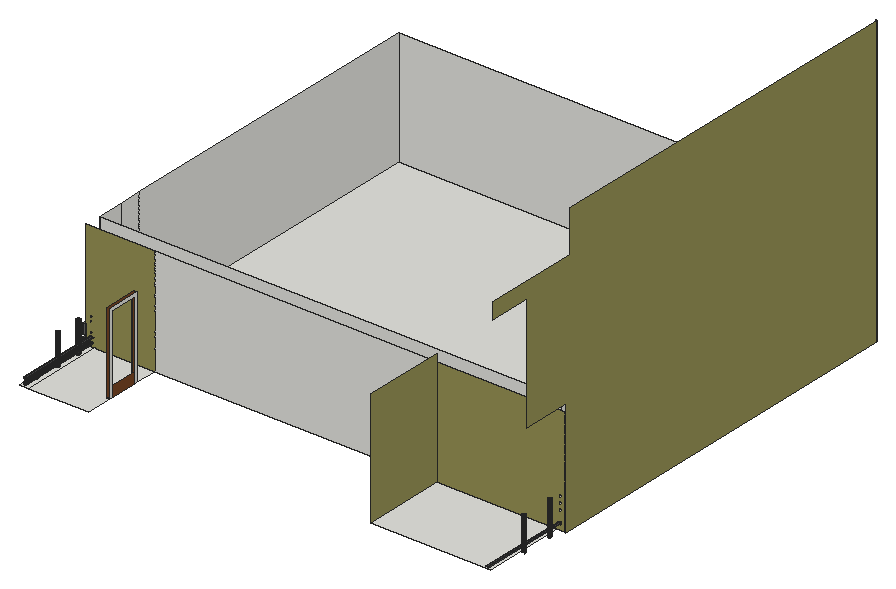
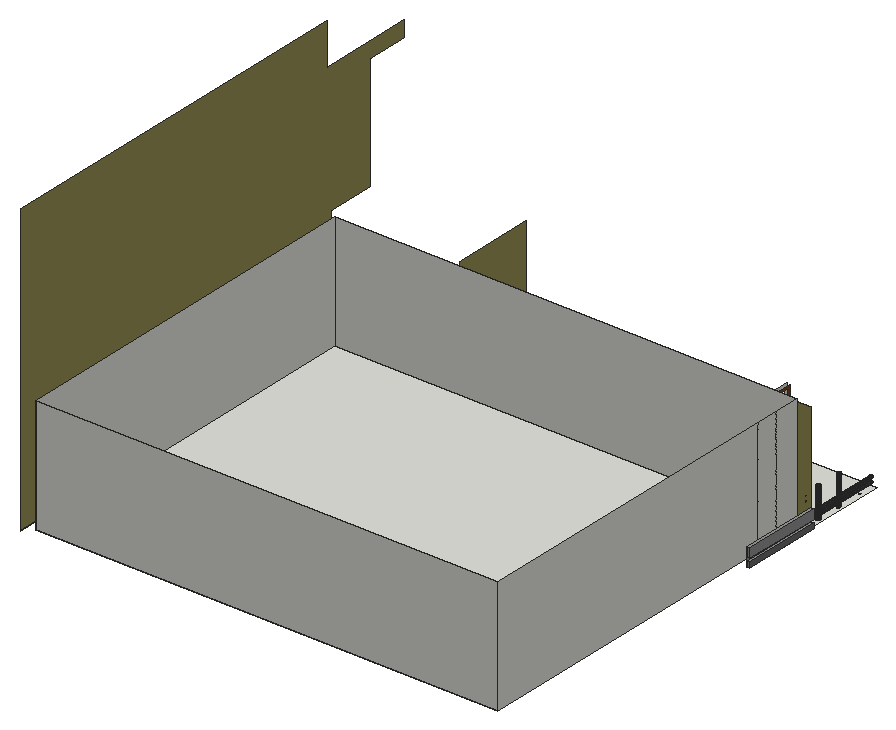
# SketchUp Ruby script. Lengths in inches.
U = 1.inch
M = Sketchup.active_model
def pt(a) = Geom::Point3d.new(a.map { |v| v * U })
def face(e, loops, mat)
  f = e.add_face(loops[0].map { |a| pt(a) })
  loops[1..].each { |l| e.add_face(l.map { |a| pt(a) }).erase! }
  f.material = f.back_material = mat if mat
  f
end
# faces: each face lists its corners as indices into pts; further lists are holes
def faces(e, pts, list, mat = nil) = list.each { |f| face(e, (f[0].is_a?(Array) ? f : [f]).map { |l| l.map { |i| pts[i] } }, mat) }
# xy, xz, yz: faces in a plane at the given z, y or x. An outline is a flat list of corners, or four numbers for a rectangle; further outlines are holes
def ring(l) = l.size == 4 ? [[l[0], l[1]], [l[2], l[1]], [l[2], l[3]], [l[0], l[3]]] : l.each_slice(2).to_a
def flat(e, list, mat, &to3) = list.each { |f| face(e, (f[0].is_a?(Array) ? f : [f]).map { |l| ring(l).map { |u, v| to3.(u, v) } }, mat) }
def xy(e, z, list, mat = nil) = flat(e, list, mat) { |x, y| [x, y, z] }
def xz(e, y, list, mat = nil) = flat(e, list, mat) { |x, z| [x, y, z] }
def yz(e, x, list, mat = nil) = flat(e, list, mat) { |y, z| [x, y, z] }
def lines(e, pts, list) = list.each { |a, b| e.add_line(pt(pts[a]), pt(pts[b])) }
# prism: a flat outline (further loops are holes) pulled along v
def prism(e, loops, v, mat = nil)
  f = face(e, loops, mat); d = Geom::Vector3d.new(v.map { |x| x * U })
  f.pushpull(f.normal.samedirection?(d) ? d.length : -d.length)
end
def box(e, o, s, mat = nil) = prism(e, [[o, [o[0] + s[0], o[1], o[2]], [o[0] + s[0], o[1] + s[1], o[2]], [o[0], o[1] + s[1], o[2]]]], [0, 0, s[2]], mat)
def at(x, y, z, deg = 0) = Geom::Transformation.translation(pt([x, y, z])) * Geom::Transformation.rotation(ORIGIN, Z_AXIS, deg.degrees)
def axes(o, x, y, z) = Geom::Transformation.new([*x, 0, *y, 0, *z, 0, *pt(o).to_a, 1])
def part(name) = M.definitions.add(name)
# library, detail: a bought-in or finely detailed component or shape, given as its bounding box
def library(name, o, s) = part(name).tap { |d| box(d.entities, o, s) }
def detail(e, o, s) = box(e.add_group.entities, o, s)
def put(e, d, t, mat = nil) = e.add_instance(d, t).tap { |i| i.material = mat if mat }
def group(e, t, mat = nil) = e.add_group.tap { |g| g.transformation = t; g.material = mat if mat }.entities
root = M.entities
M.materials.add("[0057_DarkKhaki]").color = [150, 145, 85]
M.materials.add("[0134_DimGray]").color = [105, 105, 105]
M.materials.add("[0137_Black]").color = [71, 71, 71]
M.materials.add("[Color M05]").color = [145, 145, 145]
M.materials.add("[Wood Veneer 01]").color = [120, 70, 37]
xy(root,123,[[[11.875,31.0625,20.875,116.75],[15.96,45.8,15.46,45.87,15,46.06,14.59,46.37,14.29,46.77,14.09,47.24,14.03,47.74,14.09,48.24,14.29,48.71,14.59,49.11,15,49.41,15.46,49.61,15.96,49.67,16.47,49.61,16.93,49.41,17.33,49.11,17.64,48.71,17.84,48.24,17.9,47.74,17.84,47.24,17.64,46.77,17.33,46.37,16.93,46.06,16.47,45.87],[15.96,72.86,15.46,72.93,15,73.12,14.59,73.43,14.29,73.83,14.09,74.3,14.03,74.8,14.09,75.3,14.29,75.77,14.59,76.17,15,76.48,15.46,76.67,15.96,76.74,16.47,76.67,16.93,76.48,17.33,76.17,17.64,75.77,17.84,75.3,17.9,74.8,17.84,74.3,17.64,73.83,17.33,73.43,16.93,73.12,16.47,72.93],[15.96,99.36,15.46,99.43,15,99.62,14.59,99.93,14.29,100.33,14.09,100.8,14.03,101.3,14.09,101.8,14.29,102.27,14.59,102.67,15,102.98,15.46,103.17,15.96,103.24,16.47,103.17,16.93,102.98,17.33,102.67,17.64,102.27,17.84,101.8,17.9,101.3,17.84,100.8,17.64,100.33,17.33,99.93,16.93,99.62,16.47,99.43]],[20.875,31.0625,82.85,31.0625,82.85,58.11,79.85,58.11,79.85,61.11,82.85,61.11,82.85,91.11,79.85,91.11,79.85,94.11,82.85,94.11,82.85,116.75,20.875,116.75],[376.99,31.0625,501.6875,116.75],[79.85,91.11,82.85,94.11],[509.75,116.75,510.6875,520.875],
  [20.875,122.75,501.6875,511.875]])
xy(root,123,[[8.875,116.75,11.875,150.26],[8.875,150.26,11.875,174.3],[8.875,174.3,11.875,199.5]],"[Color M05]")
xy(root,128.9,[[8.875,116.75,11.875,199.5]],"[Color M05]")
xy(root,131.94,[[8.875,116.75,11.875,199.5]],"[Color M05]")
xz(root,91.11,[[79.85,123,82.85,204]],"[Wood Veneer 01]")
xz(root,94.11,[[79.85,123,82.85,207]],"[Wood Veneer 01]")
xz(root,116.75,[[82.85,123,376.99,235.42],[509.75,123,510.6875,235.42]])
xz(root,116.75,[[[11.875,123,82.85,235.42],[17.02,125.05,16.66,125.1,16.33,125.24,16.05,125.46,15.83,125.74,15.69,126.07,15.65,126.43,15.69,126.79,15.83,127.12,16.05,127.4,16.33,127.62,16.66,127.76,17.02,127.8,17.375,127.76,17.71,127.62,17.99,127.4,18.21,127.12,18.35,126.79,18.4,126.43,18.35,126.07,18.21,125.74,17.99,125.46,17.71,125.24,17.375,125.1],[17.02,149.74,16.66,149.79,16.33,149.93,16.05,150.14,15.83,150.43,15.69,150.76,15.65,151.12,15.69,151.47,15.83,151.8,16.05,152.09,16.33,152.31,16.66,152.44,17.02,152.49,17.375,152.44,17.71,152.31,17.99,152.09,18.21,151.8,18.35,151.47,18.4,151.12,18.35,150.76,18.21,150.43,17.99,150.14,17.71,149.93,17.375,149.79],[17.02,144.8,16.66,144.85,16.33,144.99,16.05,145.21,15.83,145.49,15.69,145.82,15.65,146.18,15.69,146.54,15.83,146.87,16.05,147.15,16.33,147.37,16.66,147.51,17.02,147.55,17.375,147.51,17.71,147.37,17.99,147.15,18.21,146.87,18.35,146.54,18.4,146.18,18.35,145.82,18.21,145.49,17.99,145.21,17.71,144.99,17.375,144.85],[17.02,134.93,16.66,134.98,16.33,135.11,16.05,135.33,15.83,135.62,15.69,135.95,15.65,136.3,15.69,136.66,15.83,136.99,16.05,137.28,16.33,137.49,16.66,137.63,17.02,137.68,17.375,137.63,17.71,137.49,17.99,137.28,18.21,136.99,18.35,136.66,18.4,136.3,18.35,135.95,18.21,135.62,17.99,135.33,17.71,135.11,17.375,134.98]],[[376.99,123,509.75,235.42],[504.95,127.5625,504.46,127.625,504.01,127.8125,503.62,128.11,503.32,128.5,503.14,128.95,503.07,129.4375,503.14,129.92,503.32,130.375,503.62,130.76,504.01,131.0625,504.46,131.25,504.95,131.3125,505.43,131.25,505.88,131.0625,506.27,130.76,506.57,130.375,506.76,129.92,506.82,129.4375,506.76,128.95,506.57,128.5,506.27,128.11,505.88,127.8125,505.43,127.625],[504.95,140.4375,504.46,140.5,504.01,140.6875,503.62,140.99,503.32,141.375,503.14,141.83,503.07,142.3125,503.14,142.8,503.32,143.25,503.62,143.64,504.01,143.9375,504.46,144.12,504.95,144.1875,505.43,144.12,505.88,143.9375,506.27,143.64,506.57,143.25,506.76,142.8,506.82,142.3125,506.76,141.83,506.57,141.375,506.27,140.99,505.88,140.6875,505.43,140.5],[504.95,146.875,504.46,146.9375,504.01,147.125,503.62,147.42,503.32,147.8125,503.14,148.26,503.07,148.75,503.14,149.23,503.32,149.6875,503.62,150.08,504.01,150.375,504.46,150.56,504.95,150.625,505.43,150.56,505.88,150.375,506.27,150.08,506.57,149.6875,506.76,149.23,506.82,148.75,506.76,148.26,506.57,147.8125,506.27,147.42,505.88,147.125,505.43,146.9375],[504.95,153.3125,504.46,153.375,504.01,153.5625,503.62,153.86,503.32,154.25,503.14,154.7,503.07,155.1875,503.14,155.67,503.32,156.125,503.62,156.51,504.01,156.8125,504.46,157,504.95,157.0625,505.43,157,505.88,156.8125,506.27,156.51,506.57,156.125,506.76,155.67,506.82,155.1875,506.76,154.7,506.57,154.25,506.27,153.86,505.88,153.5625,505.43,153.375]]],"[0057_DarkKhaki]")
xz(root,116.75,[[8.875,123,11.875,128.9],[8.875,131.94,11.875,142.03]],"[0134_DimGray]")
xz(root,118.3125,[[17.02,129.99,16.66,130.04,16.33,130.18,16.05,130.39,15.83,130.68,15.69,131.01,15.65,131.37,15.69,131.72,15.83,132.05,16.05,132.34,16.33,132.56,16.66,132.69,17.02,132.74,17.375,132.69,17.71,132.56,17.99,132.34,18.21,132.05,18.35,131.72,18.4,131.37,18.35,131.01,18.21,130.68,17.99,130.39,17.71,130.18,17.375,130.04]])
xz(root,122.75,[[20.875,123,501.6875,243]])
xz(root,199.5,[[8.875,123,11.875,128.9],[8.875,131.94,11.875,142.03]],"[Color M05]")
xz(root,511.875,[[20.875,123,501.6875,243]])
xz(root,520.875,[[509.75,123,510.6875,423]])
yz(root,8.875,[[116.75,123,199.5,128.9]],"[0134_DimGray]")
yz(root,8.875,[[116.75,131.94,199.5,142.03]],"[Color M05]")
yz(root,11.875,[[116.75,123,199.5,128.9],[116.75,131.94,199.5,142.03]])
yz(root,11.875,[[116.75,128.9,199.5,131.94]],"[Color M05]")
yz(root,20.875,[[122.75,123,150.26,243],[150.26,123,174.3,243],[174.3,123,511.875,243]])
yz(root,79.85,[[58.11,123,58.11,207,94.11,207,94.11,123,91.11,123,91.11,204,61.11,204,61.11,123]],"[Wood Veneer 01]")
yz(root,82.85,[[58.11,123,61.11,123,61.11,204,91.11,204,91.11,123,94.11,123,94.11,207,58.11,207]])
yz(root,82.85,[[61.11,123,91.11,134.05]],"[Wood Veneer 01]")
yz(root,376.99,[[31.0625,123,116.75,243]],"[0057_DarkKhaki]")
yz(root,501.6875,[[122.75,123,511.875,243]])
yz(root,510.6875,[[116.75,123,520.875,123,520.875,423,122.75,423,122.75,379.43,22.0625,379.43,22.0625,363,66.25,363,66.25,243.17,116.75,243.17]],"[0057_DarkKhaki]")
p = [[502.97,69.67,123],[503.03,69.22,123],[503.03,69.22,158.25],[502.97,69.67,158.25],[506.41,69.22,123],[506.47,69.67,123],
  [506.47,69.67,158.25],[506.41,69.22,158.25],[503.03,70.125,123],[503.03,70.125,158.25],[506.41,70.125,123],[506.41,70.125,158.25],
  [503.21,70.55,123],[503.21,70.55,158.25],[506.24,70.55,123],[506.24,70.55,158.25],[503.49,70.91,123],[503.49,70.91,158.25],
  [505.96,70.91,123],[505.96,70.91,158.25],[503.85,71.1875,123],[503.85,71.1875,158.25],[505.6,71.1875,123],[505.6,71.1875,158.25],
  [504.27,71.36,123],[504.27,71.36,158.25],[505.18,71.36,123],[505.18,71.36,158.25],[504.72,71.42,123],[504.72,71.42,158.25],
  [15,73.12,123],[15.46,72.93,123],[15.46,72.93,154.6875],[15,73.12,154.6875],[15.96,72.86,123],[15.96,72.86,154.6875],
  [16.47,72.93,123],[16.47,72.93,154.6875],[16.93,73.12,123],[16.93,73.12,154.6875],[14.59,73.43,123],[14.59,73.43,154.6875],
  [17.33,73.43,123],[17.33,73.43,154.6875],[14.29,73.83,123],[14.29,73.83,154.6875],[17.64,73.83,123],[17.64,73.83,154.6875],
  [14.09,74.3,123],[14.09,74.3,154.6875],[17.84,74.3,123],[17.84,74.3,154.6875],[14.03,74.8,123],[14.03,74.8,154.6875],
  [17.9,74.8,123],[17.9,74.8,154.6875],[14.09,75.3,123],[14.09,75.3,154.6875],[17.84,75.3,123],[17.84,75.3,154.6875],
  [14.29,75.77,123],[14.29,75.77,154.6875],[17.64,75.77,123],[17.64,75.77,154.6875],[14.59,76.17,123],[14.59,76.17,154.6875],
  [17.33,76.17,123],[17.33,76.17,154.6875],[15,76.48,123],[15,76.48,154.6875],[16.93,76.48,123],[16.93,76.48,154.6875],
  [15.46,76.67,123],[15.46,76.67,154.6875],[16.47,76.67,123],[16.47,76.67,154.6875],[15.96,76.74,123],[15.96,76.74,154.6875],
  [15,99.62,123],[15.46,99.43,123],[15.46,99.43,154.75],[15,99.62,154.75],[15.96,99.36,123],[15.96,99.36,154.75],
  [16.47,99.43,123],[16.47,99.43,154.75],[16.93,99.62,123],[16.93,99.62,154.75],[14.59,99.93,123],[14.59,99.93,154.75],
  [17.33,99.93,123],[17.33,99.93,154.75],[14.29,100.33,123],[14.29,100.33,154.75],[17.64,100.33,123],[17.64,100.33,154.75],
  [14.09,100.8,123],[14.09,100.8,154.75],[17.84,100.8,123],[17.84,100.8,154.75],[14.03,101.3,123],[14.03,101.3,154.75],
  [17.9,101.3,123],[17.9,101.3,154.75],[14.09,101.8,123],[14.09,101.8,154.75],[17.84,101.8,123],[17.84,101.8,154.75],
  [14.29,102.27,123],[14.29,102.27,154.75],[17.64,102.27,123],[17.64,102.27,154.75],[503.85,102.4,123],[504.27,102.23,123],
  [504.27,102.23,158.25],[503.85,102.4,158.25],[504.72,102.17,123],[504.72,102.17,158.25],[505.18,102.23,123],[505.18,102.23,158.25],
  [505.6,102.4,123],[505.6,102.4,158.25],[14.59,102.67,123],[14.59,102.67,154.75],[17.33,102.67,123],[17.33,102.67,154.75],
  [503.49,102.68,123],[503.49,102.68,158.25],[505.96,102.68,123],[505.96,102.68,158.25],[15,102.98,123],[15,102.98,154.75],
  [16.93,102.98,123],[16.93,102.98,154.75],[503.21,103.05,123],[503.21,103.05,158.25],[506.24,103.05,123],[506.24,103.05,158.25],
  [15.46,103.17,123],[15.46,103.17,154.75],[16.47,103.17,123],[16.47,103.17,154.75],[503.03,103.47,123],[503.03,103.47,158.25],
  [506.41,103.47,123],[506.41,103.47,158.25],[15.96,103.24,123],[15.96,103.24,154.75],[502.97,103.92,123],[502.97,103.92,158.25],
  [506.47,103.92,123],[506.47,103.92,158.25],[503.03,104.375,123],[503.03,104.375,158.25],[506.41,104.375,123],[506.41,104.375,158.25],
  [503.21,104.8,123],[503.21,104.8,158.25],[506.24,104.8,123],[506.24,104.8,158.25],[503.49,105.16,123],[503.49,105.16,158.25],
  [505.96,105.16,123],[505.96,105.16,158.25],[503.85,105.4375,123],[503.85,105.4375,158.25],[505.6,105.4375,123],[505.6,105.4375,158.25],
  [504.27,105.61,123],[504.27,105.61,158.25],[505.18,105.61,123],[505.18,105.61,158.25],[504.72,105.67,123],[504.72,105.67,158.25],
  [16.66,31.0625,125.1],[16.33,31.0625,125.24],[16.33,116.75,125.24],[16.66,116.75,125.1],[17.02,31.0625,125.05],[17.02,116.75,125.05],
  [17.375,31.0625,125.1],[17.375,116.75,125.1],[17.71,31.0625,125.24],[17.71,116.75,125.24],[16.05,31.0625,125.46],[16.05,116.75,125.46],
  [17.99,31.0625,125.46],[17.99,116.75,125.46],[15.83,31.0625,125.74],[15.83,116.75,125.74],[18.21,31.0625,125.74],[18.21,116.75,125.74],
  [15.69,31.0625,126.07],[15.69,116.75,126.07],[18.35,31.0625,126.07],[18.35,116.75,126.07],[15.65,31.0625,126.43],[15.65,116.75,126.43],
  [18.4,31.0625,126.43],[18.4,116.75,126.43],[15.69,31.0625,126.79],[15.69,116.75,126.79],[18.35,31.0625,126.79],[18.35,116.75,126.79],
  [15.83,31.0625,127.12],[15.83,116.75,127.12],[18.21,31.0625,127.12],[18.21,116.75,127.12],[16.05,31.0625,127.4],[16.05,116.75,127.4],
  [17.99,31.0625,127.4],[17.99,116.75,127.4],[16.33,31.0625,127.62],[16.33,116.75,127.62],[17.71,31.0625,127.62],[17.71,116.75,127.62],
  [16.66,31.0625,127.76],[16.66,116.75,127.76],[17.375,31.0625,127.76],[17.375,116.75,127.76],[17.02,31.0625,127.8],[17.02,116.75,127.8],
  [16.66,31.0625,130.04],[16.33,31.0625,130.18],[16.33,118.3125,130.18],[16.66,118.3125,130.04],[17.02,31.0625,129.99],[17.02,118.3125,129.99],
  [17.375,31.0625,130.04],[17.375,118.3125,130.04],[17.71,31.0625,130.18],[17.71,118.3125,130.18],[16.05,31.0625,130.39],[16.05,118.3125,130.39],
  [17.99,31.0625,130.39],[17.99,118.3125,130.39],[506.27,22.0625,130.76],[506.57,22.0625,130.375],[506.57,116.75,130.375],[506.27,116.75,130.76],
  [15.83,31.0625,130.68],[15.83,118.3125,130.68],[18.21,31.0625,130.68],[18.21,118.3125,130.68],[15.69,31.0625,131.01],[15.69,118.3125,131.01],
  [18.35,31.0625,131.01],[18.35,118.3125,131.01],[503.62,22.0625,130.76],[504.01,22.0625,131.0625],[504.01,116.75,131.0625],[503.62,116.75,130.76],
  [505.88,22.0625,131.0625],[505.88,116.75,131.0625],[15.65,31.0625,131.37],[15.65,118.3125,131.37],[18.4,31.0625,131.37],[18.4,118.3125,131.37],
  [504.46,22.0625,131.25],[504.46,116.75,131.25],[505.43,22.0625,131.25],[505.43,116.75,131.25],[504.95,22.0625,131.3125],[504.95,116.75,131.3125],
  [15.69,31.0625,131.72],[15.69,118.3125,131.72],[18.35,31.0625,131.72],[18.35,118.3125,131.72],[15.83,31.0625,132.05],[15.83,118.3125,132.05],
  [18.21,31.0625,132.05],[18.21,118.3125,132.05],[16.05,31.0625,132.34],[16.05,118.3125,132.34],[17.99,31.0625,132.34],[17.99,118.3125,132.34],
  [16.33,31.0625,132.56],[16.33,118.3125,132.56],[17.71,31.0625,132.56],[17.71,118.3125,132.56],[16.66,31.0625,132.69],[16.66,118.3125,132.69],
  [17.375,31.0625,132.69],[17.375,118.3125,132.69],[17.02,31.0625,132.74],[17.02,118.3125,132.74]]
faces(root,p,[[0,1,2,3],[4,5,6,7],[8,0,3,9],[5,10,11,6],[12,8,9,13],[10,14,15,11],[16,12,13,17],[14,18,19,15],
  [20,16,17,21],[18,22,23,19],[24,20,21,25],[22,26,27,23],[28,24,25,29],[26,28,29,27],[30,31,32,33],[31,34,35,32],
  [34,36,37,35],[36,38,39,37],[40,30,33,41],[38,42,43,39],[44,40,41,45],[42,46,47,43],[48,44,45,49],[46,50,51,47],
  [52,48,49,53],[50,54,55,51],[56,52,53,57],[54,58,59,55],[60,56,57,61],[58,62,63,59],[64,60,61,65],[62,66,67,63],
  [68,64,65,69],[66,70,71,67],[72,68,69,73],[70,74,75,71],[76,72,73,77],[74,76,77,75],[78,79,80,81],[79,82,83,80],
  [82,84,85,83],[84,86,87,85],[88,78,81,89],[86,90,91,87],[92,88,89,93],[90,94,95,91],[96,92,93,97],[94,98,99,95],
  [100,96,97,101],[98,102,103,99],[104,100,101,105],[102,106,107,103],[108,104,105,109],[106,110,111,107],[112,113,114,115],[113,116,117,114],
  [116,118,119,117],[118,120,121,119],[122,108,109,123],[110,124,125,111],[126,112,115,127],[120,128,129,121],[130,122,123,131],[124,132,133,125],
  [134,126,127,135],[128,136,137,129],[138,130,131,139],[132,140,141,133],[142,134,135,143],[136,144,145,137],[146,138,139,147],[140,146,147,141],
  [148,142,143,149],[144,150,151,145],[152,148,149,153],[150,154,155,151],[156,152,153,157],[154,158,159,155],[160,156,157,161],[158,162,163,159],
  [164,160,161,165],[162,166,167,163],[168,164,165,169],[166,170,171,167],[172,168,169,173],[170,172,173,171],[174,175,176,177],[178,174,177,179],
  [180,178,179,181],[182,180,181,183],[175,184,185,176],[186,182,183,187],[184,188,189,185],[190,186,187,191],[188,192,193,189],[194,190,191,195],
  [192,196,197,193],[198,194,195,199],[196,200,201,197],[202,198,199,203],[200,204,205,201],[206,202,203,207],[204,208,209,205],[210,206,207,211],
  [208,212,213,209],[214,210,211,215],[212,216,217,213],[218,214,215,219],[216,220,221,217],[220,218,219,221],[222,223,224,225],[226,222,225,227],
  [228,226,227,229],[230,228,229,231],[223,232,233,224],[234,230,231,235],[236,237,238,239],[232,240,241,233],[242,234,235,243],[240,244,245,241],
  [246,242,243,247],[248,249,250,251],[252,236,239,253],[244,254,255,245],[256,246,247,257],[249,258,259,250],[260,252,253,261],[258,262,263,259],
  [262,260,261,263],[254,264,265,255],[266,256,257,267],[264,268,269,265],[270,266,267,271],[268,272,273,269],[274,270,271,275],[272,276,277,273],
  [278,274,275,279],[276,280,281,277],[282,278,279,283],[280,284,285,281],[284,282,283,285]],"[0137_Black]")
